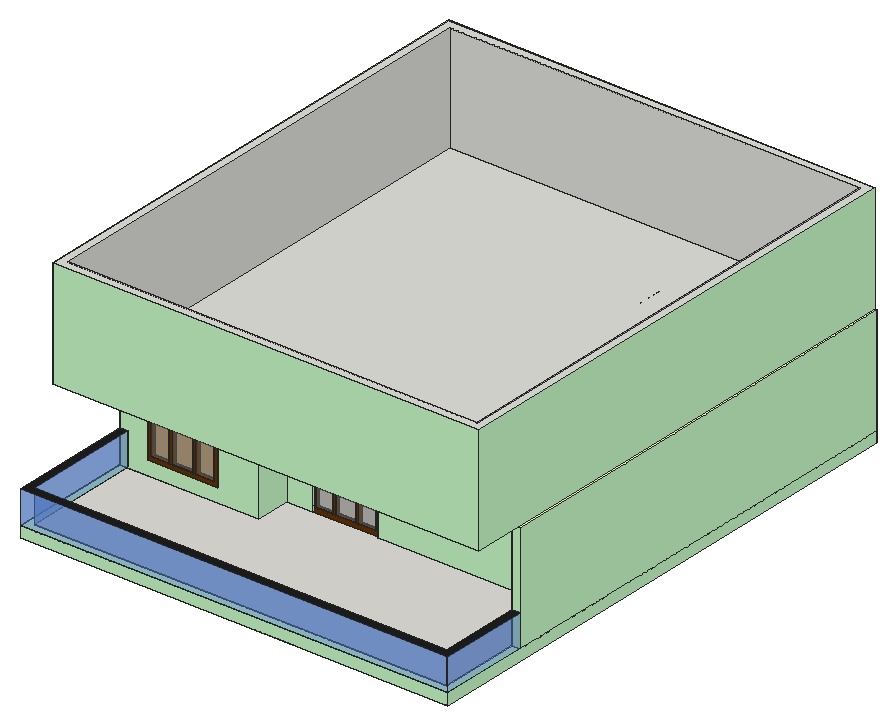
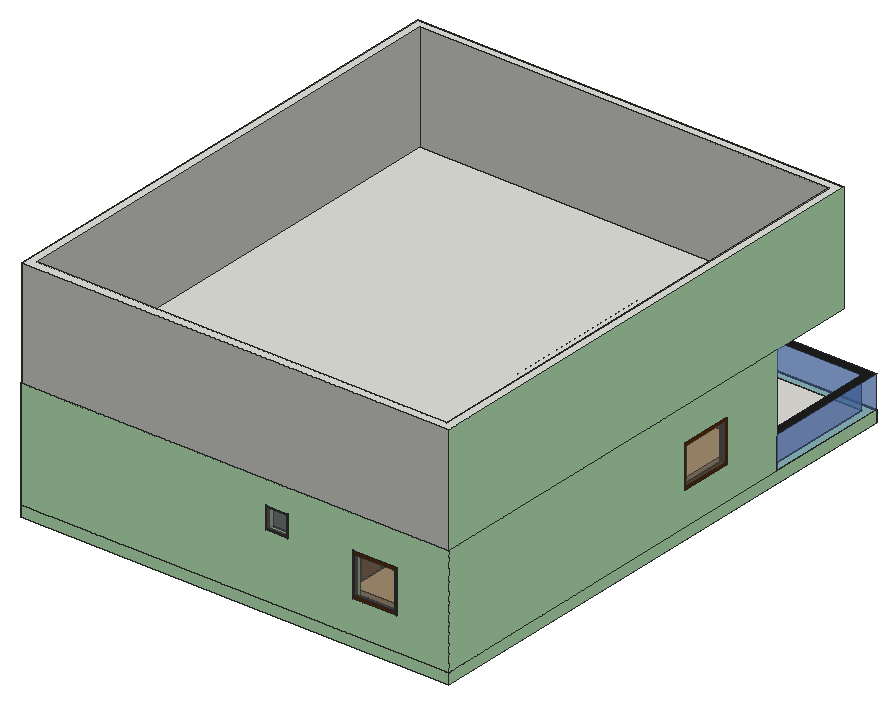
# SketchUp Ruby script. Lengths in inches.
U = 1.inch
M = Sketchup.active_model
def pt(a) = Geom::Point3d.new(a.map { |v| v * U })
def face(e, loops, mat)
  f = e.add_face(loops[0].map { |a| pt(a) })
  loops[1..].each { |l| e.add_face(l.map { |a| pt(a) }).erase! }
  f.material = f.back_material = mat if mat
  f
end
# faces: each face lists its corners as indices into pts; further lists are holes
def faces(e, pts, list, mat = nil) = list.each { |f| face(e, (f[0].is_a?(Array) ? f : [f]).map { |l| l.map { |i| pts[i] } }, mat) }
# xy, xz, yz: faces in a plane at the given z, y or x. An outline is a flat list of corners, or four numbers for a rectangle; further outlines are holes
def ring(l) = l.size == 4 ? [[l[0], l[1]], [l[2], l[1]], [l[2], l[3]], [l[0], l[3]]] : l.each_slice(2).to_a
def flat(e, list, mat, &to3) = list.each { |f| face(e, (f[0].is_a?(Array) ? f : [f]).map { |l| ring(l).map { |u, v| to3.(u, v) } }, mat) }
def xy(e, z, list, mat = nil) = flat(e, list, mat) { |x, y| [x, y, z] }
def xz(e, y, list, mat = nil) = flat(e, list, mat) { |x, z| [x, y, z] }
def yz(e, x, list, mat = nil) = flat(e, list, mat) { |y, z| [x, y, z] }
def lines(e, pts, list) = list.each { |a, b| e.add_line(pt(pts[a]), pt(pts[b])) }
# prism: a flat outline (further loops are holes) pulled along v
def prism(e, loops, v, mat = nil)
  f = face(e, loops, mat); d = Geom::Vector3d.new(v.map { |x| x * U })
  f.pushpull(f.normal.samedirection?(d) ? d.length : -d.length)
end
def box(e, o, s, mat = nil) = prism(e, [[o, [o[0] + s[0], o[1], o[2]], [o[0] + s[0], o[1] + s[1], o[2]], [o[0], o[1] + s[1], o[2]]]], [0, 0, s[2]], mat)
def at(x, y, z, deg = 0) = Geom::Transformation.translation(pt([x, y, z])) * Geom::Transformation.rotation(ORIGIN, Z_AXIS, deg.degrees)
def axes(o, x, y, z) = Geom::Transformation.new([*x, 0, *y, 0, *z, 0, *pt(o).to_a, 1])
def part(name) = M.definitions.add(name)
# library, detail: a bought-in or finely detailed component or shape, given as its bounding box
def library(name, o, s) = part(name).tap { |d| box(d.entities, o, s) }
def detail(e, o, s) = box(e.add_group.entities, o, s)
def put(e, d, t, mat = nil) = e.add_instance(d, t).tap { |i| i.material = mat if mat }
def group(e, t, mat = nil) = e.add_group.tap { |g| g.transformation = t; g.material = mat if mat }.entities
root = M.entities
M.materials.add("[Color C08]").color = [102, 51, 0]
M.materials.add("[Color E01]").color = [255, 255, 204]
M.materials.add("[Color G01]").color = [204, 255, 204]
M.materials.add("[Color K01]").color = [255, 204, 255]
M.materials.add("[Color M08]").color = [30, 30, 30]
M.materials.add("[Concrete Pavers Block Multi]").color = [124, 140, 145]
M.materials.add("[Marble Carrara Gold Floor Tile]").color = [225, 223, 217]
M.materials.add("[Resin Turquoise]").color = [117, 218, 223]
M.materials.add("[Translucent Glass Blue]").color = [100, 149, 237]
M.materials["[Translucent Glass Blue]"].alpha = 0.5
M.materials.add("[Translucent Glass Gray]").color = [128, 128, 128]
M.materials["[Translucent Glass Gray]"].alpha = 0.5
M.materials.add("[Wood Floor]").color = [155, 105, 61]
c1 = library("28",[-28.6,-106.68,0],[90.94,96.67,40.97])
c2 = part("Group\#7")
xy(c2.entities,0,[[0,0,36,6]])
xy(c2.entities,4.09,[[4.09,0,31.91,2.0625]],"[Color C08]")
xy(c2.entities,79.91,[[4.09,0,31.91,2.0625]],"[Color C08]")
xy(c2.entities,84,[[0,0,36,6]],"[Color C08]")
xz(c2.entities,0,[[[0,0,36,84],[4.09,4.09,31.91,79.91]]],"[Color C08]")
xz(c2.entities,0.25,[[26.54,38.97,27.4,39.08,28.2,39.41,28.88,39.9375,29.41,40.625,29.74,41.42,29.85,42.28,29.74,43.14,29.41,43.9375,28.88,44.625,28.2,45.15,27.4,45.48,26.54,45.59,25.68,45.48,24.89,45.15,24.2,44.625,23.67,43.9375,23.34,43.14,23.23,42.28,23.34,41.42,23.67,40.625,24.2,39.9375,24.89,39.41,25.68,39.08]],"[Color C08]")
xz(c2.entities,2.0625,[[[4.09,4.09,31.91,79.91],[26.54,38.97,25.68,39.08,24.89,39.41,24.2,39.9375,23.67,40.625,23.34,41.42,23.23,42.28,23.34,43.14,23.67,43.9375,24.2,44.625,24.89,45.15,25.68,45.48,26.54,45.59,27.4,45.48,28.2,45.15,28.88,44.625,29.41,43.9375,29.74,43.14,29.85,42.28,29.74,41.42,29.41,40.625,28.88,39.9375,28.2,39.41,27.4,39.08]]],"[Wood Floor]")
xz(c2.entities,6,[[0,0,36,84]])
yz(c2.entities,0,[[0,0,6,84]],"[Color C08]")
yz(c2.entities,4.09,[[0,4.09,2.0625,79.91]],"[Color C08]")
yz(c2.entities,31.91,[[0,4.09,2.0625,79.91]],"[Color C08]")
yz(c2.entities,36,[[0,0,6,84]],"[Color C08]")
p = [[25.68,2.0625,39.08],[26.54,2.0625,38.97],[26.54,0.25,38.97],[25.68,0.25,39.08],[27.4,2.0625,39.08],[27.4,0.25,39.08],
  [24.89,2.0625,39.41],[24.89,0.25,39.41],[28.2,2.0625,39.41],[28.2,0.25,39.41],[24.2,2.0625,39.9375],[24.2,0.25,39.9375],
  [28.88,2.0625,39.9375],[28.88,0.25,39.9375],[23.67,2.0625,40.625],[23.67,0.25,40.625],[29.41,2.0625,40.625],[29.41,0.25,40.625],
  [23.34,2.0625,41.42],[23.34,0.25,41.42],[29.74,2.0625,41.42],[29.74,0.25,41.42],[23.23,2.0625,42.28],[23.23,0.25,42.28],
  [29.85,2.0625,42.28],[29.85,0.25,42.28],[23.34,2.0625,43.14],[23.34,0.25,43.14],[29.74,2.0625,43.14],[29.74,0.25,43.14],
  [23.67,2.0625,43.9375],[23.67,0.25,43.9375],[29.41,2.0625,43.9375],[29.41,0.25,43.9375],[24.2,2.0625,44.625],[24.2,0.25,44.625],
  [28.88,2.0625,44.625],[28.88,0.25,44.625],[24.89,2.0625,45.15],[24.89,0.25,45.15],[28.2,2.0625,45.15],[28.2,0.25,45.15],
  [25.68,2.0625,45.48],[25.68,0.25,45.48],[27.4,2.0625,45.48],[27.4,0.25,45.48],[26.54,2.0625,45.59],[26.54,0.25,45.59]]
faces(c2.entities,p,[[0,1,2,3],[1,4,5,2],[6,0,3,7],[4,8,9,5],[10,6,7,11],[8,12,13,9],[14,10,11,15],[12,16,17,13],
  [18,14,15,19],[16,20,21,17],[22,18,19,23],[20,24,25,21],[26,22,23,27],[24,28,29,25],[30,26,27,31],[28,32,33,29],
  [34,30,31,35],[32,36,37,33],[38,34,35,39],[36,40,41,37],[42,38,39,43],[40,44,45,41],[46,42,43,47],[44,46,47,45]],"[Color C08]")
c3 = part("Group\#12")
xy(c3.entities,0,[[0,0,77.625,5.875]])
xy(c3.entities,3.68,[[3.68,0,23.65,0.75],[23.65,0,27.29,5.875],[27.29,0,50.21,0.75],[50.21,0,53.85,5.875],[53.85,0,73.95,0.75],
  [3.68,0.75,23.65,5.875],[27.29,0.75,50.21,5.875],[53.85,0.75,73.95,5.875]],"[Color C08]")
xy(c3.entities,68.14,[[3.68,0,23.65,0.75],[23.65,0,27.29,5.875],[27.29,0,50.21,0.75],[50.21,0,53.85,5.875],[53.85,0,73.95,0.75],
  [3.68,0.75,23.65,5.875],[27.29,0.75,50.21,5.875],[53.85,0.75,73.95,5.875]])
xy(c3.entities,71.8125,[[0,0,77.625,5.875]],"[Color C08]")
xz(c3.entities,0,[[[0,0,77.625,71.8125],[3.68,3.68,73.95,68.14]],[23.65,3.68,27.29,68.14],[50.21,3.68,53.85,68.14]],"[Color C08]")
xz(c3.entities,0.75,[[3.68,3.68,23.65,68.14],[27.29,3.68,50.21,68.14],[53.85,3.68,73.95,68.14]],"[Translucent Glass Gray]")
xz(c3.entities,5.875,[[[0,0,77.625,71.8125],[3.68,3.68,73.95,68.14]],[23.65,3.68,27.29,68.14],[50.21,3.68,53.85,68.14]],"[Color C08]")
yz(c3.entities,0,[[0,0,5.875,71.8125]],"[Color C08]")
yz(c3.entities,3.68,[[0,3.68,0.75,68.14],[0.75,3.68,5.875,68.14]],"[Color C08]")
yz(c3.entities,23.65,[[0,3.68,0.75,68.14]])
yz(c3.entities,23.65,[[0.75,3.68,5.875,68.14]],"[Color C08]")
yz(c3.entities,27.29,[[0,3.68,0.75,68.14],[0.75,3.68,5.875,68.14]],"[Color C08]")
yz(c3.entities,50.21,[[0,3.68,0.75,68.14],[0.75,3.68,5.875,68.14]],"[Color C08]")
yz(c3.entities,53.85,[[0,3.68,0.75,68.14],[0.75,3.68,5.875,68.14]],"[Color C08]")
yz(c3.entities,73.95,[[0,3.68,0.75,68.14],[0.75,3.68,5.875,68.14]],"[Color C08]")
yz(c3.entities,77.625,[[0,0,5.875,71.8125]],"[Color C08]")
c4 = part("Group\#14")
xy(c4.entities,0,[[0,0,8.11,83.5625]])
xy(c4.entities,3.3125,[[7.9,3.57,8.11,80]])
xy(c4.entities,3.3125,[[0,3.57,7.9,80]],"[Color C08]")
xy(c4.entities,44.6875,[[0,3.57,7.9,80],[7.9,3.57,8.11,80]])
xy(c4.entities,48,[[0,0,8.11,83.5625]],"[Color C08]")
xz(c4.entities,0,[[0,0,8.11,48]],"[Color C08]")
xz(c4.entities,3.57,[[7.9,3.3125,8.11,44.6875]])
xz(c4.entities,3.57,[[0,3.3125,7.9,44.6875]],"[Color C08]")
xz(c4.entities,80,[[7.9,3.3125,8.11,44.6875]])
xz(c4.entities,80,[[0,3.3125,7.9,44.6875]],"[Color C08]")
xz(c4.entities,83.5625,[[0,0,8.11,48]],"[Color C08]")
yz(c4.entities,0,[[[0,0,83.5625,48],[3.57,3.3125,80,44.6875]]],"[Color C08]")
yz(c4.entities,7.9,[[3.57,3.3125,80,44.6875]],"[Translucent Glass Gray]")
yz(c4.entities,8.11,[[[0,0,83.5625,48],[3.57,3.3125,80,44.6875]]],"[Color C08]")
c5 = part("Group\#4")
xy(c5.entities,0,[[0,0,8.11,83.5625]])
xy(c5.entities,3.3125,[[7.9,3.57,8.11,80]])
xy(c5.entities,3.3125,[[0,3.57,7.9,80]],"[Color C08]")
xy(c5.entities,44.6875,[[0,3.57,7.9,80],[7.9,3.57,8.11,80]])
xy(c5.entities,48,[[0,0,8.11,83.5625]],"[Color C08]")
xz(c5.entities,0,[[0,0,8.11,48]],"[Color C08]")
xz(c5.entities,3.57,[[7.9,3.3125,8.11,44.6875]])
xz(c5.entities,3.57,[[0,3.3125,7.9,44.6875]],"[Color C08]")
xz(c5.entities,80,[[7.9,3.3125,8.11,44.6875]])
xz(c5.entities,80,[[0,3.3125,7.9,44.6875]],"[Color C08]")
xz(c5.entities,83.5625,[[0,0,8.11,48]],"[Color C08]")
yz(c5.entities,0,[[[0,0,83.5625,48],[3.57,3.3125,80,44.6875]]],"[Color C08]")
yz(c5.entities,7.9,[[3.57,3.3125,80,44.6875]],"[Translucent Glass Gray]")
yz(c5.entities,8.11,[[[0,0,83.5625,48],[3.57,3.3125,80,44.6875]]],"[Color C08]")
xy(root,119.1875,[[311.23,460.51,311.23,490.39,312.24,492.6875,313.82,495.71,315.59,498.61,317.57,501.39,319.72,504.03,322.05,506.52,324.53,508.85,327.18,511,329.96,512.97,332.86,514.75,335.88,516.33,338.18,517.34,427,517.34,427,489.02,426.88,486.07,426.54,483.23,425.98,480.43,425.2,477.68,424.2,475.01,423,472.42,421.59,469.93,420,467.5625,418.22,465.33,416.27,463.24,414.15,461.3125,413.12,460.51]],"[Color K01]")
xy(root,119.1875,[[[320.15,22.59,320.15,26.28,346.72,26.28,346.72,58.59,320.15,58.59,320.15,133.78,287.85,133.78,287.85,58.59,178.15,58.59,178.15,226.59,133.15,226.59,133.15,283.41,159.28,283.41,160.85,292.17,163.32,300.72,166.65,308.96,170.82,316.82,175.78,324.21,181.48,331.04,187.85,337.25,194.83,342.76,202.34,347.53,210.31,351.49,218.64,354.61,227.25,356.85,251.25,356.85,251.25,386.28,277.15,386.28,277.15,568.28,449.85,568.28,449.85,410.63,407.78,410.63,407.78,368.58,418.74,368.58,418.74,309.14,418.72,309.14,418.72,268.07,418.47,262.89,417.72,257.76,416.47,252.72,414.74,247.83,412.55,243.13,409.91,238.67,406.85,234.48,403.4,230.61,399.59,227.09,395.45,223.95,391.03,221.23,386.375,218.96,371.8,218.96,371.8,170.28,449.85,170.28,449.85,58.59,405.33,58.59,405.33,26.28,449.85,26.28,449.85,22.59],[331.35,68.47,438.72,159.72],[306.15,455.42,414.86,455.42,417.43,457.42,419.84,459.62,422.07,462,424.1,464.55,425.92,467.25,427.52,470.09,428.9,473.04,430.04,476.1,430.93,479.23,431.57,482.43,431.95,485.67,432.08,488.92,432.08,522.42,337.12,522.42,333.68,520.92,330.36,519.18,327.16,517.22,324.1,515.05,321.1875,512.68,318.45,510.12,315.89,507.38,313.52,504.47,311.35,501.41,309.39,498.21,307.65,494.89,306.15,491.45],[301,168.625,307,168.625,307,183.4375,336.83,183.4375,336.83,189.4375,301,189.4375]],[[331.35,68.47,438.72,159.72],[337.55,74.67,432.52,153.52]],[[337.55,74.67,432.52,153.52],[385.83,87.07,392.91,87.83,399.57,90.4,405.33,94.6,409.81,100.15,412.69,106.67,413.8,113.71,413.04,120.8,410.47,127.45,406.27,133.21,400.72,137.69,394.21,140.58,387.16,141.68,380.07,140.93,373.42,138.36,367.66,134.16,363.18,128.61,360.29,122.09,359.1875,115.05,359.95,107.96,362.51,101.31,366.71,95.54,372.26,91.07,378.78,88.18],[421.43,136.83,422.66,137.04,423.78,137.55,424.74,138.34,425.46,139.36,425.89,140.52,426.01,141.75,425.8,142.97,425.28,144.1,424.49,145.06,423.48,145.78,422.32,146.21,421.08,146.32,419.86,146.12,418.73,145.6,417.78,144.81,417.06,143.8,416.63,142.64,416.51,141.4,416.72,140.18,417.24,139.05,418.03,138.1,419.04,137.38,420.2,136.95],[348.25,138.17,349.47,138.375,350.6,138.89,351.55,139.68,352.27,140.69,352.7,141.86,352.82,143.09,352.61,144.3125,352.1,145.44,351.31,146.4,350.29,147.11,349.13,147.55,347.9,147.66,346.68,147.45,345.55,146.9375,344.59,146.15,343.875,145.14,343.44,143.97,343.33,142.74,343.53,141.52,344.05,140.39,344.84,139.43,345.85,138.72,347.02,138.28],[348.25,81.79,349.47,82,350.6,82.52,351.55,83.31,352.27,84.32,352.7,85.48,352.82,86.72,352.61,87.9375,352.1,89.07,351.31,90.02,350.29,90.74,349.13,91.17,347.9,91.29,346.68,91.08,345.55,90.5625,344.59,89.77,343.875,88.76,343.44,87.6,343.33,86.36,343.53,85.14,344.05,84.01,344.84,83.06,345.85,82.34,347.02,81.91],[419.3125,81.79,420.53,82,421.66,82.52,422.62,83.31,423.33,84.32,423.77,85.48,423.88,86.72,423.68,87.9375,423.16,89.07,422.37,90.02,421.36,90.74,420.2,91.17,418.96,91.29,417.74,91.08,416.61,90.5625,415.66,89.77,414.9375,88.76,414.51,87.6,414.39,86.36,414.6,85.14,415.11,84.01,415.9,83.06,416.92,82.34,418.08,81.91]],[[348.25,81.79,349.47,82,350.6,82.52,351.55,83.31,352.27,84.32,352.7,85.48,352.82,86.72,352.61,87.9375,352.1,89.07,351.31,90.02,350.29,90.74,349.13,91.17,347.9,91.29,346.68,91.08,345.55,90.5625,344.59,89.77,343.875,88.76,343.44,87.6,343.33,86.36,343.53,85.14,344.05,84.01,344.84,83.06,345.85,82.34,347.02,81.91],[348.07,83.14,347.19,83.26,346.375,83.6,345.67,84.14,345.13,84.84,344.79,85.66,344.68,86.54,344.79,87.42,345.13,88.24,345.67,88.94,346.375,89.48,347.19,89.82,348.07,89.9375,348.95,89.82,349.77,89.48,350.48,88.94,351.02,88.24,351.36,87.42,351.47,86.54,351.36,85.66,351.02,84.84,350.48,84.14,349.77,83.6,348.95,83.26]],[[419.3125,81.79,420.53,82,421.66,82.52,422.62,83.31,423.33,84.32,423.77,85.48,423.88,86.72,423.68,87.9375,423.16,89.07,422.37,90.02,421.36,90.74,420.2,91.17,418.96,91.29,417.74,91.08,416.61,90.5625,415.66,89.77,414.9375,88.76,414.51,87.6,414.39,86.36,414.6,85.14,415.11,84.01,415.9,83.06,416.92,82.34,418.08,81.91],[419.14,83.14,418.26,83.26,417.4375,83.6,416.73,84.14,416.19,84.84,415.85,85.66,415.74,86.54,415.85,87.42,416.19,88.24,416.73,88.94,417.4375,89.48,418.26,89.82,419.14,89.9375,420.02,89.82,420.84,89.48,421.54,88.94,422.08,88.24,422.42,87.42,422.53,86.54,422.42,85.66,422.08,84.84,421.54,84.14,420.84,83.6,420.02,83.26]],
  [348.07,83.14,347.19,83.26,346.375,83.6,345.67,84.14,345.13,84.84,344.79,85.66,344.68,86.54,344.79,87.42,345.13,88.24,345.67,88.94,346.375,89.48,347.19,89.82,348.07,89.9375,348.95,89.82,349.77,89.48,350.48,88.94,351.02,88.24,351.36,87.42,351.47,86.54,351.36,85.66,351.02,84.84,350.48,84.14,349.77,83.6,348.95,83.26],[419.14,83.14,418.26,83.26,417.4375,83.6,416.73,84.14,416.19,84.84,415.85,85.66,415.74,86.54,415.85,87.42,416.19,88.24,416.73,88.94,417.4375,89.48,418.26,89.82,419.14,89.9375,420.02,89.82,420.84,89.48,421.54,88.94,422.08,88.24,422.42,87.42,422.53,86.54,422.42,85.66,422.08,84.84,421.54,84.14,420.84,83.6,420.02,83.26],[388.97,90.51,382.7,90.68,376.7,92.47,371.36,95.75,367.06,100.3,364.07,105.8125,362.62,111.91,362.79,118.17,364.58,124.17,367.86,129.51,372.42,133.82,377.93,136.8,384.02,138.25,390.28,138.08,396.29,136.29,401.625,133.01,405.93,128.46,408.91,122.95,410.37,116.85,410.19,110.59,408.4,104.58,405.12,99.25,400.57,94.94,395.0625,91.96],[[421.43,136.83,422.66,137.04,423.78,137.55,424.74,138.34,425.46,139.36,425.89,140.52,426.01,141.75,425.8,142.97,425.28,144.1,424.49,145.06,423.48,145.78,422.32,146.21,421.08,146.32,419.86,146.12,418.73,145.6,417.78,144.81,417.06,143.8,416.63,142.64,416.51,141.4,416.72,140.18,417.24,139.05,418.03,138.1,419.04,137.38,420.2,136.95],[421.26,138.18,420.38,138.29,419.56,138.63,418.86,139.17,418.32,139.88,417.98,140.7,417.86,141.58,417.98,142.46,418.32,143.28,418.86,143.98,419.56,144.52,420.38,144.86,421.26,144.97,422.14,144.86,422.96,144.52,423.66,143.98,424.2,143.28,424.54,142.46,424.66,141.58,424.54,140.7,424.2,139.88,423.66,139.17,422.96,138.63,422.14,138.29]],[[348.25,138.17,349.47,138.375,350.6,138.89,351.55,139.68,352.27,140.69,352.7,141.86,352.82,143.09,352.61,144.3125,352.1,145.44,351.31,146.4,350.29,147.11,349.13,147.55,347.9,147.66,346.68,147.45,345.55,146.9375,344.59,146.15,343.875,145.14,343.44,143.97,343.33,142.74,343.53,141.52,344.05,140.39,344.84,139.43,345.85,138.72,347.02,138.28],[348.07,139.52,347.19,139.63,346.375,139.97,345.67,140.51,345.13,141.22,344.79,142.04,344.68,142.91,344.79,143.79,345.13,144.61,345.67,145.32,346.375,145.86,347.19,146.2,348.07,146.3125,348.95,146.2,349.77,145.86,350.48,145.32,351.02,144.61,351.36,143.79,351.47,142.91,351.36,142.04,351.02,141.22,350.48,140.51,349.77,139.97,348.95,139.63]],
  [421.26,138.18,420.38,138.29,419.56,138.63,418.86,139.17,418.32,139.88,417.98,140.7,417.86,141.58,417.98,142.46,418.32,143.28,418.86,143.98,419.56,144.52,420.38,144.86,421.26,144.97,422.14,144.86,422.96,144.52,423.66,143.98,424.2,143.28,424.54,142.46,424.66,141.58,424.54,140.7,424.2,139.88,423.66,139.17,422.96,138.63,422.14,138.29],[348.07,139.52,347.19,139.63,346.375,139.97,345.67,140.51,345.13,141.22,344.79,142.04,344.68,142.91,344.79,143.79,345.13,144.61,345.67,145.32,346.375,145.86,347.19,146.2,348.07,146.3125,348.95,146.2,349.77,145.86,350.48,145.32,351.02,144.61,351.36,143.79,351.47,142.91,351.36,142.04,351.02,141.22,350.48,140.51,349.77,139.97,348.95,139.63],[133.15,283.41,159.28,283.41,160.85,292.17,163.32,300.72,166.65,308.96,170.82,316.82,175.78,324.21,181.48,331.04,187.85,337.25,194.83,342.76,202.34,347.53,210.31,351.49,218.64,354.61,227.25,356.85,251.25,356.85,251.25,386.28,133.15,386.28],[433.17,309.14,434.49,368.58],[448.92,309.14,449.85,368.58]],"[Marble Carrara Gold Floor Tile]")
xy(root,120,[[[0,0,9,0,9,581,120,581,120,405,9,405,9,207,159,207,159,0,165,0,165,39,301,39,301,0,307,0,307,39,463,39,463,0,472,0,472,590,0,590],[165,45,165,213,120,213,120,399,264,399,264,412.4,258,412.4,258,405,126,405,126,581,258,581,258,481.74,264,481.74,264,581,463,581,463,397.04,420.9375,397.04,420.9375,381.29,463,381.29,463,189,301,189,301,45],[307,45,463,183],[18,303,114,399],[18,213,114,297]],[9,0,159,207],[165,0,301,39],[307,0,463,39],[165,45,301,45,301,189,463,189,463,381.29,420.9375,381.29,420.9375,397.04,463,397.04,463,581,264,581,264,481.74,258,481.74,258,581,126,581,126,405,258,405,258,412.4,264,412.4,264,399,120,399,120,213,165,213],
  [18,213,114,297],[18,303,114,399],[9,405,120,581]],"[Color G01]")
xy(root,120,[[[307,9.4375,463,9.4375,463,39.4375,418.48,39.4375,418.48,45.4375,463,45.4375,463,183.4375,396.83,183.4375,396.83,189.4375,463,189.4375,463,381.73,420.9375,381.73,420.9375,397.48,463,397.48,463,581.4375,264,581.4375,264,399.4375,120,399.4375,120,213.4375,165,213.4375,165,45.4375,301,45.4375,301,120.625,307,120.625,307,45.4375,333.57,45.4375,333.57,39.4375,307,39.4375],[301,168.625,301,189.4375,336.83,189.4375,336.83,183.4375,307,183.4375,307,168.625]]],"[Marble Carrara Gold Floor Tile]")
xy(root,132,[[0,0,0,137.1875,9,137.1875,9,9,463,9,463,99.27,472,99.27,472,0],[463,99.27,463,175.9375,254.03,175.9375,254.03,181.9375,463,181.9375,463,407,451.9,407,451.9,413,463,413,463,581,200.85,581,200.85,590,472,590,472,99.27],[0,137.1875,0,265.6,9,265.6,9,143.1875,107.91,143.1875,107.91,137.1875],[107.91,137.1875,107.91,143.1875,147,143.1875,147,255.87,153,255.87,153,181.9375,182.03,181.9375,182.03,175.9375,153,175.9375,153,137.1875],[0,265.6,0,590,105.31,590,105.31,581,9,581,9,413,147,413,147,419.45,153,419.45,153,291.87,147,291.87,147,314.1875,90.95,314.1875,90.95,320.1875,147,320.1875,147,407,9,407,9,320.1875,34.9,320.1875,34.9,314.1875,9,314.1875,9,265.6],
  [229.5,407,229.5,477,153,477,153,455.45,147,455.45,147,494.61,153,494.61,153,483,229.5,483,229.5,581,235.5,581,235.5,497,307,497,307,413,408.93,413,408.93,407,295.62,407,295.62,413,301,413,301,491,235.5,491,235.5,413,259.62,413,259.62,407],[235.5,413,301,491],[147,530.61,147,581,105.31,581,105.31,590,200.85,590,200.85,581,153,581,153,530.61]],"[Color G01]")
xy(root,132,[[9,9,463,9,463,175.9375,254.03,175.9375,254.03,181.9375,463,181.9375,463,407,451.9,407,451.9,413,463,413,463,581,235.5,581,235.5,497,307,497,307,413,408.93,413,408.93,407,295.62,407,295.62,413,259.62,413,259.62,407,229.5,407,229.5,477,153,477,153,455.45,147,455.45,147,494.61,153,494.61,153,483,229.5,483,229.5,581,153,581,153,530.61,147,530.61,147,581,9,581,9,413,147,413,147,419.45,153,419.45,153,291.87,147,291.87,147,314.1875,90.95,314.1875,90.95,320.1875,147,320.1875,147,407,9,407,9,320.1875,34.9,320.1875,34.9,314.1875,9,314.1875,9,143.1875,147,143.1875,147,255.87,153,255.87,153,181.9375,182.03,181.9375,182.03,175.9375,153,175.9375,153,137.1875,9,137.1875]],"[Marble Carrara Gold Floor Tile]")
xy(root,147.35,[[31.12,137.1875,107.91,143.1875]],"[Color G01]")
xy(root,168,[[0,204.39,9,265.6],[57.31,581,105.31,590]],"[Color G01]")
xy(root,168,[[0,0,472,0,472,99.27,463,99.27,463,9,9,9,9,137.1875,0,137.1875]],"[Color M08]")
xy(root,201.9375,[[176.85,581,200.85,590]],"[Color G01]")
xy(root,216,[[0,204.39,9,265.6],[147,255.87,153,291.87],[34.9,314.1875,90.95,320.1875],[259.62,407,295.62,413],[408.93,407,451.9,413],
  [147,419.45,153,455.45],[147,494.61,153,530.61],[57.31,581,105.31,590]],"[Color G01]")
xy(root,226.76,[[176.85,581,200.85,590]],"[Color G01]")
xy(root,228,[[182.03,175.9375,254.03,181.9375]],"[Color G01]")
xy(root,228.8125,[[31.12,137.1875,107.91,143.1875]],"[Color G01]")
xy(root,252,[[0,44.5625,470.125,590]])
xy(root,252,[[[463,99.27,472,99.27,472,590,0,590,0,137.1875,153,137.1875,153,175.9375,463,175.9375],[153,181.9375,153,477,229.5,477,229.5,407,463,407,463,181.9375],[307,413,307,497,235.5,497,235.5,581,229.5,581,229.5,483,153,483,153,581,463,581,463,413],[9,143.1875,147,314.1875],[9,413,147,581],[9,320.1875,147,407],[235.5,413,301,491]]],"[Color E01]")
xy(root,253.4375,[[9,53.5625,461.125,581]])
xy(root,372,[[[0,44.5625,470.125,590],[9,53.5625,461.125,581]]])
xz(root,0,[[0,120,472,132]],"[Color G01]")
xz(root,0,[[0,132,472,168]],"[Translucent Glass Blue]")
xz(root,9,[[9,132,463,168]],"[Translucent Glass Blue]")
xz(root,44.5625,[[0,252,470.125,372]],"[Color G01]")
xz(root,53.5625,[[9,253.4375,461.125,372]])
xz(root,99.27,[[463,132,472,168],[463,168,472,252]],"[Color G01]")
xz(root,137.1875,[[0,132,9,168],[[9,132,153,132,153,252,0,252,0,168,9,168],[31.12,147.35,107.91,228.8125]]],"[Color G01]")
xz(root,143.1875,[[[9,132,147,252],[31.12,147.35,107.91,228.8125]]],"[Resin Turquoise]")
xz(root,168.625,[[301,119.1875,307,120]],"[Marble Carrara Gold Floor Tile]")
xz(root,175.9375,[[153,132,182.03,132,182.03,228,254.03,228,254.03,132,463,132,463,252,153,252]],"[Color G01]")
xz(root,181.9375,[[153,132,153,252,463,252,463,132,254.03,132,254.03,228,182.03,228,182.03,132]],"[Color E01]")
xz(root,183.4375,[[307,119.1875,336.83,120]],"[Marble Carrara Gold Floor Tile]")
xz(root,189.4375,[[301,119.1875,336.83,120]],"[Marble Carrara Gold Floor Tile]")
xz(root,204.39,[[0,168,9,216]],"[Color G01]")
xz(root,255.87,[[147,132,153,216]],"[Color G01]")
xz(root,265.6,[[0,168,9,216]],"[Color G01]")
xz(root,291.87,[[147,132,153,216]],"[Color G01]")
xz(root,314.1875,[[9,132,34.9,132,34.9,216,90.95,216,90.95,132,147,132,147,252,9,252]],"[Resin Turquoise]")
xz(root,320.1875,[[9,132,9,252,147,252,147,132,90.95,132,90.95,216,34.9,216,34.9,132]],"[Color G01]")
xz(root,407,[[9,132,147,252],[229.5,132,259.62,132,259.62,216,295.62,216,295.62,132,408.93,132,408.93,216,451.9,216,451.9,132,463,132,463,252,229.5,252]],"[Color E01]")
xz(root,413,[[9,132,147,252]],"[Color E01]")
xz(root,413,[[235.5,132,235.5,252,301,252,301,132,295.62,132,295.62,216,259.62,216,259.62,132]],"[Concrete Pavers Block Multi]")
xz(root,413,[[307,132,307,252,463,252,463,132,451.9,132,451.9,216,408.93,216,408.93,132]],"[Resin Turquoise]")
xz(root,419.45,[[147,132,153,216]],"[Color G01]")
xz(root,455.45,[[147,132,153,216]],"[Color G01]")
xz(root,477,[[153,132,229.5,252]],"[Color E01]")
xz(root,483,[[153,132,229.5,252]],"[Concrete Pavers Block Multi]")
xz(root,491,[[235.5,132,301,252]],"[Concrete Pavers Block Multi]")
xz(root,494.61,[[147,132,153,216]],"[Color G01]")
xz(root,497,[[235.5,132,307,252]],"[Resin Turquoise]")
xz(root,530.61,[[147,132,153,216]],"[Color G01]")
xz(root,581,[[9,253.4375,461.125,372]])
xz(root,581,[[[9,132,147,252],[57.31,168,105.31,216]]],"[Color E01]")
xz(root,581,[[229.5,132,235.5,252]],"[Color G01]")
xz(root,581,[[[153,132,229.5,252],[176.85,201.9375,200.85,226.76]]],"[Concrete Pavers Block Multi]")
xz(root,581,[[235.5,132,463,252]],"[Resin Turquoise]")
xz(root,590,[[0,252,470.125,372]])
xz(root,590,[[0,120,472,132],[[0,132,472,252],[57.31,168,105.31,216],[176.85,201.9375,200.85,226.76]]],"[Color G01]")
yz(root,0,[[0,120,590,132],[[137.1875,132,590,252],[204.39,168,265.6,216]],[44.5625,252,590,372]],"[Color G01]")
yz(root,0,[[0,132,137.1875,168]],"[Translucent Glass Blue]")
yz(root,9,[[53.5625,253.4375,581,372]])
yz(root,9,[[320.1875,132,407,252],[413,132,581,252]],"[Color E01]")
yz(root,9,[[[143.1875,132,314.1875,252],[204.39,168,265.6,216]]],"[Resin Turquoise]")
yz(root,9,[[9,132,137.1875,168]],"[Translucent Glass Blue]")
yz(root,31.12,[[137.1875,147.35,143.1875,228.8125]],"[Color G01]")
yz(root,34.9,[[314.1875,132,320.1875,216]],"[Color G01]")
yz(root,57.31,[[581,168,590,216]],"[Color G01]")
yz(root,90.95,[[314.1875,132,320.1875,216]],"[Color G01]")
yz(root,105.31,[[581,168,590,216]],"[Color G01]")
yz(root,107.91,[[137.1875,147.35,143.1875,228.8125]],"[Color G01]")
yz(root,147,[[320.1875,132,407,252],[413,132,413,252,581,252,581,132,530.61,132,530.61,216,494.61,216,494.61,132,455.45,132,455.45,216,419.45,216,419.45,132]],"[Color E01]")
yz(root,147,[[143.1875,132,143.1875,252,314.1875,252,314.1875,132,291.87,132,291.87,216,255.87,216,255.87,132]],"[Resin Turquoise]")
yz(root,153,[[181.9375,132,255.87,132,255.87,216,291.87,216,291.87,132,419.45,132,419.45,216,455.45,216,455.45,132,477,132,477,252,181.9375,252]],"[Color E01]")
yz(root,153,[[137.1875,132,175.9375,252],[483,132,494.61,252]],"[Color G01]")
yz(root,153,[[530.61,132,581,132,581,252,494.61,252,494.61,216,530.61,216]],"[Concrete Pavers Block Multi]")
yz(root,176.85,[[581,201.9375,590,204],[581,204,590,226.76]],"[Color G01]")
yz(root,182.03,[[175.9375,132,181.9375,137.68],[175.9375,137.68,181.9375,228]],"[Color G01]")
yz(root,200.85,[[581,201.9375,590,226.76]],"[Color G01]")
yz(root,229.5,[[407,132,477,252]],"[Color E01]")
yz(root,229.5,[[483,132,581,252]],"[Concrete Pavers Block Multi]")
yz(root,235.5,[[413,132,491,252]],"[Concrete Pavers Block Multi]")
yz(root,235.5,[[497,132,581,252]],"[Resin Turquoise]")
yz(root,254.03,[[175.9375,132,181.9375,228]],"[Color G01]")
yz(root,259.62,[[407,132,413,216]],"[Color G01]")
yz(root,295.62,[[407,132,413,216]],"[Color G01]")
yz(root,301,[[413,132,491,252]],"[Concrete Pavers Block Multi]")
yz(root,301,[[168.625,119.1875,189.4375,120]],"[Marble Carrara Gold Floor Tile]")
yz(root,307,[[168.625,119.1875,183.4375,120]],"[Marble Carrara Gold Floor Tile]")
yz(root,307,[[413,132,497,252]],"[Resin Turquoise]")
yz(root,336.83,[[183.4375,119.1875,189.4375,120]],"[Marble Carrara Gold Floor Tile]")
yz(root,408.93,[[407,132,413,216]],"[Color G01]")
yz(root,451.9,[[407,132,413,216]],"[Color G01]")
yz(root,461.125,[[53.5625,253.4375,581,372]])
yz(root,463,[[181.9375,132,407,252]],"[Color E01]")
yz(root,463,[[99.27,132,175.9375,252]],"[Color G01]")
yz(root,463,[[413,132,581,252]],"[Resin Turquoise]")
yz(root,463,[[9,132,99.27,168]],"[Translucent Glass Blue]")
yz(root,470.125,[[44.5625,252,590,372]],"[Color G01]")
yz(root,472,[[0,120,590,132],[99.27,132,590,252]],"[Color G01]")
yz(root,472,[[0,132,99.27,168]],"[Translucent Glass Blue]")
p = [[408.93,413,216],[408.93,415.375,216]]
lines(root,p,[[0,1]])
put(root,c1,at(50.9375,591.01,132))
put(root,c1,at(-1.01,195.0625,132,90))
put(root,c1,at(473.01,530.66,132,-90))
put(root,c2,axes([408.93,407,132],[1.19343,0,0],[0,0.56,0],[0,0,1]))
put(root,c2,axes([259.62,407,132],[1,0,0],[0,0.43999,0],[0,0,1]))
put(root,c2,axes([147,530.61,132],[0,-1,0],[0.43999,0,0],[0,0,1]))
put(root,c2,axes([153,255.87,132],[0,1,0],[-0.56,0,0],[0,0,1]))
put(root,c2,axes([153,419.45,132],[0,1,0],[-0.56,0,0],[0,0,1]))
put(root,c3,axes([181.58,176.48,132],[0.9333,0,0],[0,0.7476,0],[0,0,1.33681]))
put(root,c3,axes([31.12,136.99,147.35],[0.98929,0,0],[0,0.84,0],[0,0,1.12292]))
put(root,c4,axes([5.21,265.6,168],[-0.6424,0,0],[0,-0.73246,0],[0,0,1]))
put(root,c5,axes([105.31,587.08,168],[0,0.36,0],[-0.57442,0,0],[0,0,0.9864]))
put(root,c5,axes([200.85,588.1,201.9375],[0,0.234,0],[-0.28721,0,0],[0,0,0.51724]))
